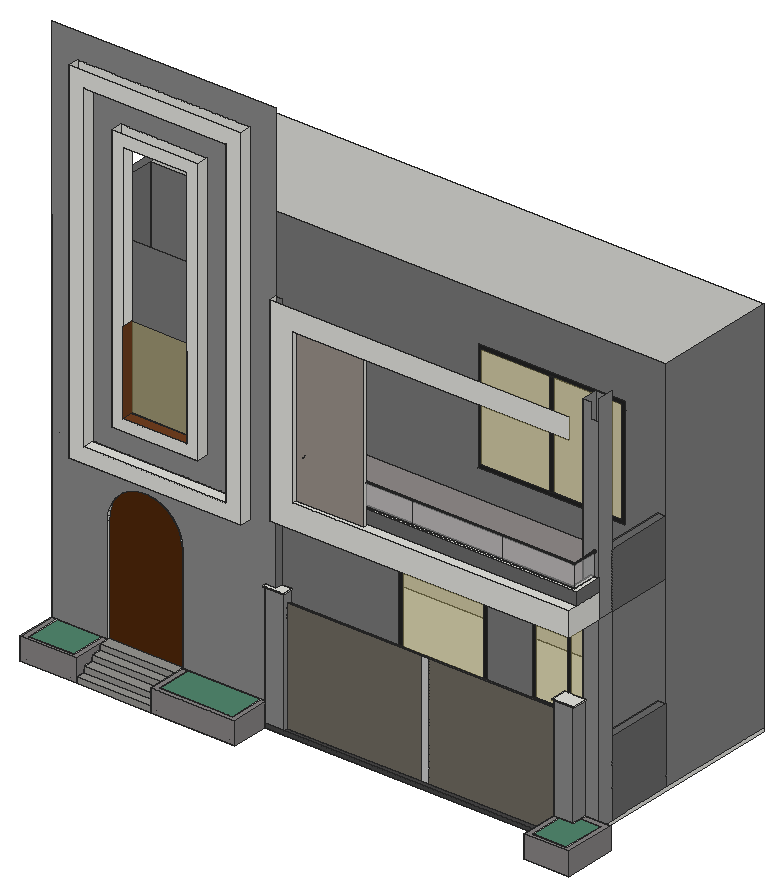
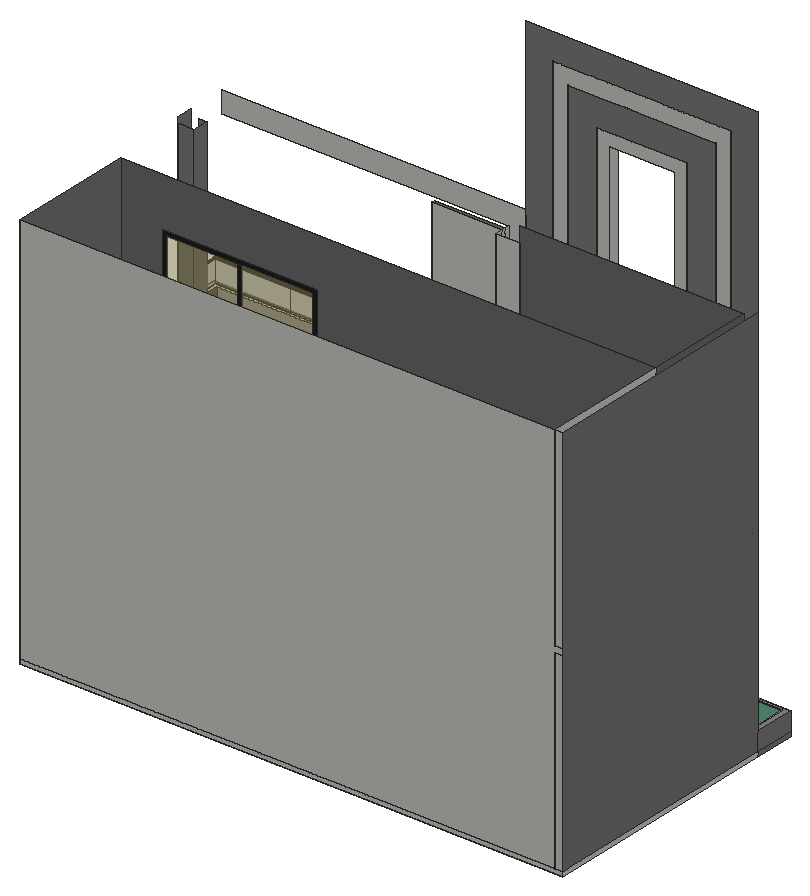
# SketchUp Ruby script. Lengths in inches.
U = 1.inch
M = Sketchup.active_model
def pt(a) = Geom::Point3d.new(a.map { |v| v * U })
def face(e, loops, mat)
  f = e.add_face(loops[0].map { |a| pt(a) })
  loops[1..].each { |l| e.add_face(l.map { |a| pt(a) }).erase! }
  f.material = f.back_material = mat if mat
  f
end
# faces: each face lists its corners as indices into pts; further lists are holes
def faces(e, pts, list, mat = nil) = list.each { |f| face(e, (f[0].is_a?(Array) ? f : [f]).map { |l| l.map { |i| pts[i] } }, mat) }
# xy, xz, yz: faces in a plane at the given z, y or x. An outline is a flat list of corners, or four numbers for a rectangle; further outlines are holes
def ring(l) = l.size == 4 ? [[l[0], l[1]], [l[2], l[1]], [l[2], l[3]], [l[0], l[3]]] : l.each_slice(2).to_a
def flat(e, list, mat, &to3) = list.each { |f| face(e, (f[0].is_a?(Array) ? f : [f]).map { |l| ring(l).map { |u, v| to3.(u, v) } }, mat) }
def xy(e, z, list, mat = nil) = flat(e, list, mat) { |x, y| [x, y, z] }
def xz(e, y, list, mat = nil) = flat(e, list, mat) { |x, z| [x, y, z] }
def yz(e, x, list, mat = nil) = flat(e, list, mat) { |y, z| [x, y, z] }
def lines(e, pts, list) = list.each { |a, b| e.add_line(pt(pts[a]), pt(pts[b])) }
# prism: a flat outline (further loops are holes) pulled along v
def prism(e, loops, v, mat = nil)
  f = face(e, loops, mat); d = Geom::Vector3d.new(v.map { |x| x * U })
  f.pushpull(f.normal.samedirection?(d) ? d.length : -d.length)
end
def box(e, o, s, mat = nil) = prism(e, [[o, [o[0] + s[0], o[1], o[2]], [o[0] + s[0], o[1] + s[1], o[2]], [o[0], o[1] + s[1], o[2]]]], [0, 0, s[2]], mat)
def at(x, y, z, deg = 0) = Geom::Transformation.translation(pt([x, y, z])) * Geom::Transformation.rotation(ORIGIN, Z_AXIS, deg.degrees)
def axes(o, x, y, z) = Geom::Transformation.new([*x, 0, *y, 0, *z, 0, *pt(o).to_a, 1])
def part(name) = M.definitions.add(name)
# library, detail: a bought-in or finely detailed component or shape, given as its bounding box
def library(name, o, s) = part(name).tap { |d| box(d.entities, o, s) }
def detail(e, o, s) = box(e.add_group.entities, o, s)
def put(e, d, t, mat = nil) = e.add_instance(d, t).tap { |i| i.material = mat if mat }
def group(e, t, mat = nil) = e.add_group.tap { |g| g.transformation = t; g.material = mat if mat }.entities
root = M.entities
M.materials.add("[0043_SaddleBrown]").color = [79, 39, 10]
M.materials.add("[0132_LightGray]").color = [137, 137, 137]
M.materials.add("[0133_Gray]").color = [128, 128, 128]
M.materials.add("[0134_DimGray]").color = [105, 105, 105]
M.materials.add("[0136_Charcoal]").color = [35, 35, 35]
M.materials.add("[Brick Tumbled]").color = [135, 132, 132]
M.materials.add("[Carrera Marble]").color = [119, 119, 119]
M.materials.add("[Cladding Stucco White]").color = [200, 200, 200]
M.materials.add("[Cladding Weathered]").color = [111, 105, 96]
M.materials.add("[Diamond Stripes]").color = [153, 144, 137]
M.materials.add("[Granite Dark Gray]").color = [69, 68, 68]
M.materials.add("[Granite Light Gray]").color = [149, 148, 144]
M.materials.add("[Stone Marble]").color = [143, 138, 136]
M.materials.add("[Translucent Glass Gray]").color = [191, 177, 107]
M.materials["[Translucent Glass Gray]"].alpha = 0.5
M.materials.add("[Translucent Glass Gray]1").color = [211, 211, 211]
M.materials["[Translucent Glass Gray]1"].alpha = 0.5
M.materials.add("[Vegetation Ivy Hedera]").color = [81, 134, 109]
M.materials.add("[Wood Cherry Original]").color = [112, 63, 31]
M.materials.add("[Wood Veneer 01]").color = [120, 70, 37]
xy(root,0,[[12,0,192,126],[192,0,432,18],[432,0,702,126],[1629.1875,0,1629.1875,119,1647.1875,119,1647.1875,12,1755.1875,12,1755.1875,149,1692,149,1692,167,1773.1875,167,1773.1875,0],[1647.1875,12,1647.1875,119,1692,119,1692,149,1755.1875,149,1755.1875,12],
  [192,18,432,126],[702,119,702,126,12,126,12,882,1692,882,1692,119]])
xy(root,12,[[30,12,174,126],[450,12,684,126],[1629.1875,119,1692,167],[1666.59,167,1692,222],[1641.1875,222,1692,272.8125],
  [1666.59,272.8125,1692,492],[36,492,1692,882]])
xy(root,12,[[762,119,1629.1875,133.21],[762,133.21,1629.1875,141.23],[762,141.23,1629.1875,141.23,1629.1875,167,1666.59,167,1666.59,222,1641.1875,222,1641.1875,272.8125,1666.59,272.8125,1666.59,492,36,492,36,150,762,150]],"[Granite Dark Gray]")
xy(root,18,[[192,0,432,29.875]],"[Granite Light Gray]")
xy(root,36,[[192,29.875,432,62.5625]],"[Granite Light Gray]")
xy(root,53.25,[[1647.1875,12,1647.1875,119,1692,119,1692,149,1755.1875,149,1755.1875,12]])
xy(root,54,[[192,62.5625,432,94.28]],"[Granite Light Gray]")
xy(root,72,[[12,0,192,0,192,126,174,126,174,12,30,12,30,126,12,126],[432,0,702,0,702,126,684,126,684,12,450,12,450,126,432,126],[1629.1875,0,1773.1875,0,1773.1875,167,1692,167,1692,149,1755.1875,149,1755.1875,12,1647.1875,12,1647.1875,119,1629.1875,119]],"[Brick Tumbled]")
xy(root,72,[[192,94.28,432,132]],"[Granite Light Gray]")
xy(root,72,[[30,12,174,126],[450,12,684,126],[1647.1875,12,1755.1875,12,1755.1875,149,1692,149,1692,119,1647.1875,119]],"[Vegetation Ivy Hedera]")
xy(root,252,[[1666.59,272.8125,1692,492]],"[0134_DimGray]")
xy(root,372,[[762,133.21,1629.1875,141.23]],"[Granite Dark Gray]")
xy(root,405,[[699,116,699,126,702,126,702,119,762,119,762,150,765,150,765,116],[1626.1875,116,1626.1875,167,1629.1875,167,1629.1875,119,1692,119,1692,167,1695,167,1695,116]])
xy(root,408,[[699,116,765,116,765,150,732,150,732,126,699,126],[1626.1875,116,1695,167]])
xy(root,576,[[96,90,648,126]])
xy(root,612,[[824.34,185.95,818.08,186.17,812.09,188,806.77,191.32,802.5,195.9,799.56,201.43,798.15,207.53,798.36,213.8,800.19,219.79,803.51,225.1,808.09,229.375,813.625,232.32,819.73,233.73,825.99,233.51,831.98,231.68,837.3,228.36,841.57,223.78,844.51,218.25,845.92,212.15,845.71,205.88,843.88,199.89,840.56,194.58,835.98,190.3,830.45,187.36],[1112.34,185.95,1106.08,186.17,1100.09,188,1094.77,191.32,1090.5,195.9,1087.56,201.43,1086.15,207.53,1086.36,213.8,1088.19,219.79,1091.51,225.1,1096.09,229.375,1101.625,232.32,1107.73,233.73,1113.99,233.51,1119.98,231.68,1125.3,228.36,1129.57,223.78,1132.51,218.25,1133.92,212.15,1133.71,205.88,1131.88,199.89,1128.56,194.58,1123.98,190.3,1118.45,187.36],[1400.34,185.95,1394.08,186.17,1388.09,188,1382.77,191.32,1378.5,195.9,1375.56,201.43,1374.15,207.53,1374.36,213.8,1376.19,219.79,1379.51,225.1,1384.09,229.375,1389.625,232.32,1395.73,233.73,1401.99,233.51,1407.98,231.68,1413.3,228.36,1417.57,223.78,1420.51,218.25,1421.92,212.15,1421.71,205.88,1419.88,199.89,1416.56,194.58,1411.98,190.3,1406.45,187.36],[824.34,353.95,818.08,354.17,812.09,356,806.77,359.32,802.5,363.9,799.56,369.43,798.15,375.53,798.36,381.8,800.19,387.79,803.51,393.1,808.09,397.375,813.625,400.32,819.73,401.73,825.99,401.51,831.98,399.68,837.3,396.36,841.57,391.78,844.51,386.25,845.92,380.15,845.71,373.88,843.88,367.89,840.56,362.58,835.98,358.3,830.45,355.36],[1112.34,353.95,1106.08,354.17,1100.09,356,1094.77,359.32,1090.5,363.9,1087.56,369.43,1086.15,375.53,1086.36,381.8,1088.19,387.79,1091.51,393.1,1096.09,397.375,1101.625,400.32,1107.73,401.73,1113.99,401.51,1119.98,399.68,1125.3,396.36,1129.57,391.78,1132.51,386.25,1133.92,380.15,1133.71,373.88,1131.88,367.89,1128.56,362.58,1123.98,358.3,1118.45,355.36],
  [1400.34,353.95,1394.08,354.17,1388.09,356,1382.77,359.32,1378.5,363.9,1375.56,369.43,1374.15,375.53,1374.36,381.8,1376.19,387.79,1379.51,393.1,1384.09,397.375,1389.625,400.32,1395.73,401.73,1401.99,401.51,1407.98,399.68,1413.3,396.36,1417.57,391.78,1420.51,386.25,1421.92,380.15,1421.71,373.88,1419.88,367.89,1416.56,362.58,1411.98,358.3,1406.45,355.36]])
xy(root,612,[[[732,102,732,150,36,150,36,492,1692,492,1692,272.8125,1641.1875,272.8125,1641.1875,222,1692,222,1692,102],[1112.34,353.95,1118.45,355.36,1123.98,358.3,1128.56,362.58,1131.88,367.89,1133.71,373.88,1133.92,380.15,1132.51,386.25,1129.57,391.78,1125.3,396.36,1119.98,399.68,1113.99,401.51,1107.73,401.73,1101.625,400.32,1096.09,397.375,1091.51,393.1,1088.19,387.79,1086.36,381.8,1086.15,375.53,1087.56,369.43,1090.5,363.9,1094.77,359.32,1100.09,356,1106.08,354.17],[1400.34,353.95,1406.45,355.36,1411.98,358.3,1416.56,362.58,1419.88,367.89,1421.71,373.88,1421.92,380.15,1420.51,386.25,1417.57,391.78,1413.3,396.36,1407.98,399.68,1401.99,401.51,1395.73,401.73,1389.625,400.32,1384.09,397.375,1379.51,393.1,1376.19,387.79,1374.36,381.8,1374.15,375.53,1375.56,369.43,1378.5,363.9,1382.77,359.32,1388.09,356,1394.08,354.17],[824.34,185.95,830.45,187.36,835.98,190.3,840.56,194.58,843.88,199.89,845.71,205.88,845.92,212.15,844.51,218.25,841.57,223.78,837.3,228.36,831.98,231.68,825.99,233.51,819.73,233.73,813.625,232.32,808.09,229.375,803.51,225.1,800.19,219.79,798.36,213.8,798.15,207.53,799.56,201.43,802.5,195.9,806.77,191.32,812.09,188,818.08,186.17],[824.34,353.95,830.45,355.36,835.98,358.3,840.56,362.58,843.88,367.89,845.71,373.88,845.92,380.15,844.51,386.25,841.57,391.78,837.3,396.36,831.98,399.68,825.99,401.51,819.73,401.73,813.625,400.32,808.09,397.375,803.51,393.1,800.19,387.79,798.36,381.8,798.15,375.53,799.56,369.43,802.5,363.9,806.77,359.32,812.09,356,818.08,354.17],[1112.34,185.95,1118.45,187.36,1123.98,190.3,1128.56,194.58,1131.88,199.89,1133.71,205.88,1133.92,212.15,1132.51,218.25,1129.57,223.78,1125.3,228.36,1119.98,231.68,1113.99,233.51,1107.73,233.73,1101.625,232.32,1096.09,229.375,1091.51,225.1,1088.19,219.79,1086.36,213.8,1086.15,207.53,1087.56,201.43,1090.5,195.9,1094.77,191.32,1100.09,188,1106.08,186.17],[1400.34,185.95,1406.45,187.36,1411.98,190.3,1416.56,194.58,1419.88,199.89,1421.71,205.88,1421.92,212.15,1420.51,218.25,1417.57,223.78,1413.3,228.36,1407.98,231.68,1401.99,233.51,1395.73,233.73,1389.625,232.32,1384.09,229.375,1379.51,225.1,1376.19,219.79,1374.36,213.8,1374.15,207.53,1375.56,201.43,1378.5,195.9,1382.77,191.32,1388.09,188,1394.08,186.17]]],"[Wood Veneer 01]")
xy(root,624,[[144,90,600,126]])
xy(root,630,[[36,150,1666.59,150,1666.59,222,1641.1875,222,1641.1875,272.8125,1666.59,272.8125,1666.59,492,36,492]],"[Stone Marble]")
xy(root,690,[[804,102,1692,102,1692,133,804,133,804,126,1021.625,126,1021.625,115.125,804,115.125],[804,115.125,1021.625,126],[732,126,804,150]])
xy(root,712.57,[[232.57,90,511.43,126]])
xy(root,732,[[804,133,1692,133,1692,222,1679.3,222,1679.3,141.5,804,141.5],[804,141.5,1679.3,141.5,1679.3,222,1666.59,222,1666.59,150,804,150]])
xy(root,748.57,[[268.57,90,475.43,126]],"[Wood Cherry Original]")
xy(root,792,[[1666.59,272.8125,1692,492]],"[0134_DimGray]")
xz(root,0,[[12,0,192,72],[432,0,702,72],[1629.1875,0,1773.1875,72]],"[Brick Tumbled]")
xz(root,0,[[192,0,432,18]],"[Granite Light Gray]")
xz(root,12,[[1647.1875,0,1755.1875,53.25],[30,12,174,72],[450,12,684,72],[1647.1875,53.25,1755.1875,72]])
xz(root,29.875,[[192,18,432,36]],"[Granite Light Gray]")
xz(root,62.5625,[[192,36,432,54]],"[Granite Light Gray]")
xz(root,90,[[[96,576,648,1704],[144,624,600,1656]],[[232.57,712.57,511.43,1567.43],[268.57,748.57,475.43,1531.43]]])
xz(root,94.28,[[192,54,432,72]],"[Granite Light Gray]")
xz(root,102,[[732,612,1692,612,1692,690,804,690,804,1182,1692,1182,1692,1248,732,1248]])
xz(root,115.125,[[804,690,1021.625,1182]],"[Diamond Stripes]")
xz(root,116,[[699,405,765,408],[1626.1875,405,1695,408]])
xz(root,119,[[1629.1875,0,1647.1875,12],[1647.1875,0,1692,12],[1629.1875,12,1647.1875,72],[1647.1875,12,1692,53.25],[1647.1875,53.25,1692,72]])
xz(root,119,[[702,12,762,405],[1629.1875,72,1692,405]],"[0132_LightGray]")
xz(root,119,[[702,0,1629.1875,12]],"[Granite Dark Gray]")
xz(root,126,[[12,0,12,72,30,72,30,12,174,12,174,72,192,72,192,0],[192,0,432,18],[432,0,432,72,450,72,450,12,684,12,684,72,702,72,702,0],[30,12,36,72],[36,12,174,72],
  [450,12,684,72],[192,18,432,36],[192,36,432,54],[699,405,702,408],[[96,576,648,1704],[144,624,600,1656]],
  [804,690,1021.625,1182],[[232.57,712.57,511.43,1567.43],[268.57,748.57,475.43,1531.43]]])
xz(root,126,[[[12,72,192,72,192,412.67,193.01,428.18,196.01,443.44,200.96,458.17,207.78,472.15,216.34,485.12,226.51,496.88,238.12,507.23,250.97,515.98,264.84,523.01,279.55,528,285.88,529.79,292.34,531.04,298.86,531.94,305.42,532.49,312,532.67,318.58,532.49,325.14,531.94,331.66,531.04,338.12,529.79,344.45,528,359.16,523.01,373.03,515.98,385.88,507.23,397.49,496.88,407.66,485.12,416.22,472.15,423.04,458.17,427.99,443.44,430.99,428.18,432,412.67,432,72,702,72,702,405,699,405,699,408,732,408,732,1788,12,1788],[96,576,648,1704]],[[144,624,600,1656],[232.57,712.57,511.43,1567.43]]],"[0132_LightGray]")
xz(root,126,[[268.57,748.57,475.43,1012.57]],"[Translucent Glass Gray]")
xz(root,132,[[192,72,432,72,432,412.67,430.99,428.18,427.99,443.44,423.04,458.17,416.22,472.15,407.66,485.12,397.49,496.88,385.88,507.23,373.03,515.98,359.16,523.01,344.45,528,338.12,529.79,331.66,531.04,325.14,531.94,318.58,532.49,312,532.67,305.42,532.49,298.86,531.94,292.34,531.04,285.88,529.79,279.55,528,264.84,523.01,250.97,515.98,238.12,507.23,226.51,496.88,216.34,485.12,207.78,472.15,200.96,458.17,196.01,443.44,193.01,428.18,192,412.67]],"[0043_SaddleBrown]")
xz(root,133,[[804,690,1692,732]],"[0134_DimGray]")
xz(root,133.21,[[1195.59,12,1216.73,372]],"[Cladding Stucco White]")
xz(root,133.21,[[762,12,1195.59,372],[1216.73,12,1629.1875,372]],"[Cladding Weathered]")
xz(root,141.23,[[762,12,1629.1875,372]],"[Cladding Weathered]")
xz(root,141.5,[[804,801,1679.3,804]])
xz(root,141.5,[[804,732,1158.38,801],[1158.38,732,1446.38,801],[1446.38,732,1679.3,801]],"[Translucent Glass Gray]1")
xz(root,149,[[1692,0,1755.1875,53.25],[1692,53.25,1755.1875,72]])
xz(root,150,[[762,405,765,408],[732,630,732,690,804,690,804,732,1666.59,732,1666.59,630],[732,690,804,1182]])
xz(root,150,[[732,12,762,408]],"[0132_LightGray]")
xz(root,150,[[36,12,732,612],[36,630,732,1230]],"[Carrera Marble]")
xz(root,167,[[1692,0,1773.1875,72],[1626.1875,405,1629.1875,408],[1692,405,1695,408]])
xz(root,167,[[1629.1875,12,1692,408]],"[0132_LightGray]")
xz(root,222,[[1666.59,630,1692,690],[1666.59,690,1692,732],[1679.3,801,1678.98,801.02,1678.67,801.07,1678.37,801.15,1678.08,801.26,1677.8,801.4,1677.53,801.57,1677.29,801.77,1677.07,801.99,1676.87,802.24,1676.7,802.5,1676.56,802.78,1676.44,803.07,1676.36,803.375,1676.3125,803.6875,1676.3,804,1676.3125,804.3125,1676.36,804.625,1676.44,804.93,1676.56,805.22,1676.7,805.5,1676.87,805.76,1677.07,806.01,1677.29,806.23,1677.53,806.43,1677.8,806.6,1678.08,806.74,1678.37,806.85,1678.67,806.93,1678.98,806.98,1679.3,807,1679.61,806.98,1679.92,806.93,1680.22,806.85,1680.52,806.74,1680.8,806.6,1681.06,806.43,1681.3,806.23,1681.53,806.01,1681.72,805.76,1681.89,805.5,1682.04,805.22,1682.15,804.93,1682.23,804.625,1682.28,804.3125,1682.3,804,1682.28,803.6875,1682.23,803.375,1682.15,803.07,1682.04,802.78,1681.89,802.5,1681.72,802.24,1681.53,801.99,1681.3,801.77,1681.06,801.57,1680.8,801.4,1680.52,801.26,1680.22,801.15,1679.92,801.07,1679.61,801.02]])
xz(root,222,[[1641.1875,12,1692,612],[[1641.1875,630,1666.59,630,1666.59,732,1692,732,1692,1182,1666.59,1182,1666.59,1230,1641.1875,1230],[1679.3,801,1678.98,801.02,1678.67,801.07,1678.37,801.15,1678.08,801.26,1677.8,801.4,1677.53,801.57,1677.29,801.77,1677.07,801.99,1676.87,802.24,1676.7,802.5,1676.56,802.78,1676.44,803.07,1676.36,803.375,1676.3125,803.6875,1676.3,804,1676.3125,804.3125,1676.36,804.625,1676.44,804.93,1676.56,805.22,1676.7,805.5,1676.87,805.76,1677.07,806.01,1677.29,806.23,1677.53,806.43,1677.8,806.6,1678.08,806.74,1678.37,806.85,1678.67,806.93,1678.98,806.98,1679.3,807,1679.61,806.98,1679.92,806.93,1680.22,806.85,1680.52,806.74,1680.8,806.6,1681.06,806.43,1681.3,806.23,1681.53,806.01,1681.72,805.76,1681.89,805.5,1682.04,805.22,1682.15,804.93,1682.23,804.625,1682.28,804.3125,1682.3,804,1682.28,803.6875,1682.23,803.375,1682.15,803.07,1682.04,802.78,1681.89,802.5,1681.72,802.24,1681.53,801.99,1681.3,801.77,1681.06,801.57,1680.8,801.4,1680.52,801.26,1680.22,801.15,1679.92,801.07,1679.61,801.02]]],"[0132_LightGray]")
xz(root,272.8125,[[1666.59,12,1692,252],[1666.59,630,1692,732],[1666.59,732,1692,792]])
xz(root,272.8125,[[1641.1875,12,1641.1875,612,1692,612,1692,252,1666.59,252,1666.59,12],[1641.1875,630,1641.1875,1230,1692,1230,1692,792,1666.59,792,1666.59,630]],"[0132_LightGray]")
xz(root,492,[[1666.59,12,1692,252],[1666.59,630,1692,732],[1666.59,732,1692,792]])
xz(root,492,[[[831.57,12,1120.32,419.6875],[846.31,26.74,1105.58,404.95]],[[1261.8,110.58,1499.8,416.95],[1273.8,122.58,1374.8,404.95],[1386.8,122.58,1487.8,404.95]],[[1086.33,718.2,1561.39,1076.45],[1098.33,730.2,1549.39,1064.45]],[1317.86,730.2,1329.86,1064.45]],"[0136_Charcoal]")
xz(root,492,[[[36,12,831.57,12,831.57,419.6875,1120.32,419.6875,1120.32,12,1666.59,12,1666.59,252,1692,252,1692,612,36,612],[1261.8,110.58,1499.8,416.95]],[[36,630,1666.59,630,1666.59,792,1692,792,1692,1230,36,1230],[1086.33,718.2,1561.39,1076.45]]],"[Carrera Marble]")
xz(root,492,[[846.31,26.74,1105.58,404.95],[1273.8,122.58,1374.8,404.95],[1386.8,122.58,1487.8,404.95],[1098.33,730.2,1317.86,1064.45],[1329.86,730.2,1549.39,1064.45]],"[Translucent Glass Gray]")
xz(root,882,[[12,0,1692,12],[12,12,36,612],[36,12,36,612,12,612,12,630,36,630,36,1230,1692,1230,1692,12],[12,630,36,1230]])
yz(root,12,[[126,0,882,12]])
yz(root,12,[[126,12,882,1230]],"[0133_Gray]")
yz(root,12,[[0,0,126,12],[0,12,126,72]],"[Brick Tumbled]")
yz(root,30,[[12,12,126,72]])
yz(root,36,[[492,12,882,612],[492,630,882,1230]])
yz(root,36,[[150,12,492,612],[150,630,492,1230]],"[Carrera Marble]")
yz(root,96,[[90,576,126,1704]])
yz(root,144,[[90,624,126,1656]])
yz(root,174,[[12,12,126,72]])
yz(root,192,[[0,0,126,18],[29.875,18,126,36],[62.5625,36,126,54],[94.28,54,126,72],[126,72,132,412.67]])
yz(root,192,[[0,18,29.875,18,29.875,36,62.5625,36,62.5625,54,94.28,54,94.28,72,0,72]],"[Brick Tumbled]")
yz(root,232.57,[[90,712.57,126,1567.43]])
yz(root,268.57,[[90,748.57,126,1012.57]],"[Wood Cherry Original]")
yz(root,432,[[0,0,126,18],[29.875,18,126,36],[62.5625,36,126,54],[94.28,54,126,72],[126,72,132,412.67]])
yz(root,432,[[0,18,0,72,94.28,72,94.28,54,62.5625,54,62.5625,36,29.875,36,29.875,18]],"[Brick Tumbled]")
yz(root,450,[[12,12,126,72]])
yz(root,475.43,[[90,748.57,126,1012.57]],"[Wood Cherry Original]")
yz(root,511.43,[[90,712.57,126,1567.43]])
yz(root,600,[[90,624,126,1656]])
yz(root,648,[[90,576,126,1704]])
yz(root,684,[[12,12,126,72]])
yz(root,699,[[116,405,119,408],[119,405,126,408]])
yz(root,702,[[119,0,126,72],[119,72,126,405]])
yz(root,702,[[0,0,119,72]],"[Brick Tumbled]")
yz(root,732,[[102,612,126,1248],[126,630,150,690],[126,690,150,1182]])
yz(root,732,[[126,408,150,612]],"[Carrera Marble]")
yz(root,762,[[119,12,133.21,12,133.21,372,141.23,372,141.23,12,150,12,150,405,119,405]],"[0132_LightGray]")
yz(root,762,[[133.21,12,141.23,372]],"[Granite Dark Gray]")
yz(root,765,[[116,405,150,408]])
yz(root,804,[[102,690,115.125,1182],[115.125,690,126,1182],[[126,690,133,690,133,732,150,732,150,1182,126,1182],[141.5,801,141.1875,801.02,140.875,801.07,140.57,801.15,140.28,801.26,140,801.4,139.74,801.57,139.49,801.77,139.27,801.99,139.07,802.24,138.9,802.5,138.76,802.78,138.65,803.07,138.57,803.375,138.52,803.6875,138.5,804,138.52,804.3125,138.57,804.625,138.65,804.93,138.76,805.22,138.9,805.5,139.07,805.76,139.27,806.01,139.49,806.23,139.74,806.43,140,806.6,140.28,806.74,140.57,806.85,140.875,806.93,141.1875,806.98,141.5,807,141.8125,806.98,142.125,806.93,142.43,806.85,142.72,806.74,143,806.6,143.26,806.43,143.51,806.23,143.73,806.01,143.93,805.76,144.1,805.5,144.24,805.22,144.35,804.93,144.43,804.625,144.48,804.3125,144.5,804,144.48,803.6875,144.43,803.375,144.35,803.07,144.24,802.78,144.1,802.5,143.93,802.24,143.73,801.99,143.51,801.77,143.26,801.57,143,801.4,142.72,801.26,142.43,801.15,142.125,801.07,141.8125,801.02]],[133,690,150,732]])
yz(root,1021.625,[[115.125,690,126,1182]])
yz(root,1626.1875,[[116,405,167,408]])
yz(root,1629.1875,[[119,12,119,405,167,405,167,12,141.23,12,141.23,372,133.21,372,133.21,12]],"[0132_LightGray]")
yz(root,1629.1875,[[0,0,119,72]],"[Brick Tumbled]")
yz(root,1629.1875,[[133.21,12,141.23,372]],"[Granite Dark Gray]")
yz(root,1641.1875,[[222,12,272.8125,612],[222,630,272.8125,1230]],"[0132_LightGray]")
yz(root,1647.1875,[[12,0,119,53.25],[12,53.25,119,72]])
yz(root,1666.59,[[272.8125,12,492,252],[150,630,222,732],[272.8125,630,492,792]],"[0134_DimGray]")
yz(root,1679.3,[[141.5,801,222,804]])
yz(root,1679.3,[[141.5,732,222,801]],"[Translucent Glass Gray]1")
yz(root,1692,[[119,0,149,12],[149,0,167,12],[167,0,882,12],[119,12,149,53.25],[149,12,167,72],
  [119,53.25,149,72],[102,612,222,690]])
yz(root,1692,[[222,12,272.8125,612],[119,72,167,405],[222,612,272.8125,1248]],"[0132_LightGray]")
yz(root,1692,[[492,12,882,1230]],"[0133_Gray]")
yz(root,1692,[[272.8125,12,492,252],[272.8125,612,492,792],[133,690,222,732]],"[0134_DimGray]")
yz(root,1695,[[116,405,167,408]])
yz(root,1755.1875,[[12,0,149,53.25],[12,53.25,149,72]])
yz(root,1773.1875,[[0,0,167,72]],"[Brick Tumbled]")
p = [[193.01,126,428.18],[192,126,412.67],[192,132,412.67],[193.01,132,428.18],[432,126,412.67],[430.99,126,428.18],
  [430.99,132,428.18],[432,132,412.67],[196.01,126,443.44],[196.01,132,443.44],[427.99,126,443.44],[427.99,132,443.44],
  [200.96,126,458.17],[200.96,132,458.17],[423.04,126,458.17],[423.04,132,458.17],[207.78,126,472.15],[207.78,132,472.15],
  [416.22,126,472.15],[416.22,132,472.15],[216.34,126,485.12],[216.34,132,485.12],[407.66,126,485.12],[407.66,132,485.12],
  [226.51,126,496.88],[226.51,132,496.88],[397.49,126,496.88],[397.49,132,496.88],[238.12,126,507.23],[238.12,132,507.23],
  [385.88,126,507.23],[385.88,132,507.23],[250.97,126,515.98],[250.97,132,515.98],[373.03,126,515.98],[373.03,132,515.98],
  [264.84,126,523.01],[264.84,132,523.01],[359.16,126,523.01],[359.16,132,523.01],[279.55,126,528],[279.55,132,528],
  [344.45,126,528],[344.45,132,528],[285.88,126,529.79],[285.88,132,529.79],[338.12,126,529.79],[338.12,132,529.79],
  [292.34,126,531.04],[292.34,132,531.04],[331.66,126,531.04],[331.66,132,531.04],[298.86,126,531.94],[298.86,132,531.94],
  [325.14,126,531.94],[325.14,132,531.94],[305.42,126,532.49],[305.42,132,532.49],[318.58,126,532.49],[318.58,132,532.49],
  [312,126,532.67],[312,132,532.67],[1679.61,141.1875,801.02],[1679.92,140.875,801.07],[804,140.875,801.07],[804,141.1875,801.02],
  [1679.61,222,801.02],[1679.92,222,801.07],[1679.3,141.5,801],[804,141.5,801],[1158.38,141.5,801],[1446.38,141.5,801],
  [1679.3,222,801],[1678.98,141.8125,801.02],[804,141.8125,801.02],[1678.98,222,801.02],[1678.67,142.125,801.07],[804,142.125,801.07],
  [1678.67,222,801.07],[1680.22,140.57,801.15],[1680.52,140.28,801.26],[804,140.28,801.26],[804,140.57,801.15],[1680.22,222,801.15],
  [1680.52,222,801.26],[1678.37,142.43,801.15],[804,142.43,801.15],[1678.37,222,801.15],[1678.08,142.72,801.26],[804,142.72,801.26],
  [1678.08,222,801.26],[1680.8,140,801.4],[804,140,801.4],[1680.8,222,801.4],[1677.8,143,801.4],[804,143,801.4],
  [1677.8,222,801.4],[1681.06,139.74,801.57],[804,139.74,801.57],[1681.06,222,801.57],[1677.53,143.26,801.57],[804,143.26,801.57],
  [1677.53,222,801.57],[1681.3,139.49,801.77],[804,139.49,801.77],[1681.3,222,801.77],[1677.29,143.51,801.77],[804,143.51,801.77],
  [1677.29,222,801.77],[1681.53,139.27,801.99],[804,139.27,801.99],[1681.53,222,801.99],[1677.07,143.73,801.99],[804,143.73,801.99],
  [1677.07,222,801.99],[1681.72,139.07,802.24],[804,139.07,802.24],[1681.72,222,802.24],[1676.87,143.93,802.24],[804,143.93,802.24],
  [1676.87,222,802.24],[1681.89,138.9,802.5],[804,138.9,802.5],[1681.89,222,802.5],[1676.7,144.1,802.5],[804,144.1,802.5],
  [1676.7,222,802.5],[1682.04,138.76,802.78],[804,138.76,802.78],[1682.04,222,802.78],[1676.56,144.24,802.78],[804,144.24,802.78],
  [1676.56,222,802.78],[1682.15,138.65,803.07],[804,138.65,803.07],[1682.15,222,803.07],[1676.44,144.35,803.07],[804,144.35,803.07],
  [1676.44,222,803.07],[1682.23,138.57,803.375],[804,138.57,803.375],[1682.23,222,803.375],[1676.36,144.43,803.375],[804,144.43,803.375],
  [1676.36,222,803.375],[1682.28,138.52,803.6875],[804,138.52,803.6875],[1682.28,222,803.6875],[1676.3125,144.48,803.6875],[804,144.48,803.6875],
  [1676.3125,222,803.6875],[1682.3,138.5,804],[804,138.5,804],[1682.3,222,804],[1676.3,144.5,804],[804,144.5,804],
  [1676.3,222,804],[1682.28,138.52,804.3125],[804,138.52,804.3125],[1682.28,222,804.3125],[1676.3125,144.48,804.3125],[804,144.48,804.3125],
  [1676.3125,222,804.3125],[1682.23,138.57,804.625],[804,138.57,804.625],[1682.23,222,804.625],[1676.36,144.43,804.625],[804,144.43,804.625],
  [1676.36,222,804.625],[1682.15,138.65,804.93],[804,138.65,804.93],[1682.15,222,804.93],[1676.44,144.35,804.93],[804,144.35,804.93],
  [1676.44,222,804.93],[1682.04,138.76,805.22],[804,138.76,805.22],[1682.04,222,805.22],[1676.56,144.24,805.22],[804,144.24,805.22],
  [1676.56,222,805.22],[1681.89,138.9,805.5],[804,138.9,805.5],[1681.89,222,805.5],[1676.7,144.1,805.5],[804,144.1,805.5],
  [1676.7,222,805.5],[1681.72,139.07,805.76],[804,139.07,805.76],[1681.72,222,805.76],[1676.87,143.93,805.76],[804,143.93,805.76],
  [1676.87,222,805.76],[1681.53,139.27,806.01],[804,139.27,806.01],[1681.53,222,806.01],[1677.07,143.73,806.01],[804,143.73,806.01],
  [1677.07,222,806.01],[1681.3,139.49,806.23],[804,139.49,806.23],[1681.3,222,806.23],[1677.29,143.51,806.23],[804,143.51,806.23],
  [1677.29,222,806.23],[1681.06,139.74,806.43],[804,139.74,806.43],[1681.06,222,806.43],[1677.53,143.26,806.43],[804,143.26,806.43],
  [1677.53,222,806.43],[1680.8,140,806.6],[804,140,806.6],[1680.8,222,806.6],[1677.8,143,806.6],[804,143,806.6],
  [1677.8,222,806.6],[1680.52,140.28,806.74],[804,140.28,806.74],[1680.52,222,806.74],[1678.08,142.72,806.74],[804,142.72,806.74],
  [1678.08,222,806.74],[1680.22,140.57,806.85],[804,140.57,806.85],[1680.22,222,806.85],[1678.37,142.43,806.85],[804,142.43,806.85],
  [1678.37,222,806.85],[1679.92,140.875,806.93],[804,140.875,806.93],[1679.92,222,806.93],[1679.61,141.1875,806.98],[804,141.1875,806.98],
  [1679.61,222,806.98],[1678.98,141.8125,806.98],[1678.67,142.125,806.93],[804,142.125,806.93],[804,141.8125,806.98],[1678.98,222,806.98],
  [1678.67,222,806.93],[1679.3,141.5,807],[804,141.5,807],[1679.3,222,807],[36,126,12],[36,150,12],
  [36,126,612],[36,150,612],[36,150,630],[12,150,630],[804,133,688.5625],[804,126,688.5625],
  [1692,133,688.5625],[804,133,690],[732,126,12],[732,150,12],[450,12,12],[450,0,12],
  [684,12,12],[684,0,12],[174,12,12],[174,0,12],[30,12,12],[30,0,12]]
faces(root,p,[[0,1,2,3],[4,5,6,7],[8,0,3,9],[5,10,11,6],[12,8,9,13],[10,14,15,11],[16,12,13,17],[14,18,19,15],
  [20,16,17,21],[18,22,23,19],[24,20,21,25],[22,26,27,23],[28,24,25,29],[26,30,31,27],[32,28,29,33],[30,34,35,31],
  [36,32,33,37],[34,38,39,35],[40,36,37,41],[38,42,43,39],[44,40,41,45],[42,46,47,43],[48,44,45,49],[46,50,51,47],
  [52,48,49,53],[50,54,55,51],[56,52,53,57],[54,58,59,55],[60,56,57,61],[58,60,61,59],[62,63,64,65],[66,67,63,62],
  [68,62,65,69,70,71],[72,66,62,68],[73,68,71,70,69,74],[75,72,68,73],[76,73,74,77],[78,75,73,76],[79,80,81,82],[83,84,80,79],
  [63,79,82,64],[67,83,79,63],[85,76,77,86],[87,78,76,85],[88,85,86,89],[90,87,85,88],[80,91,92,81],[84,93,91,80],
  [94,88,89,95],[96,90,88,94],[91,97,98,92],[93,99,97,91],[100,94,95,101],[102,96,94,100],[97,103,104,98],[99,105,103,97],
  [106,100,101,107],[108,102,100,106],[103,109,110,104],[105,111,109,103],[112,106,107,113],[114,108,106,112],[109,115,116,110],[111,117,115,109],
  [118,112,113,119],[120,114,112,118],[115,121,122,116],[117,123,121,115],[124,118,119,125],[126,120,118,124],[121,127,128,122],[123,129,127,121],
  [130,124,125,131],[132,126,124,130],[127,133,134,128],[129,135,133,127],[136,130,131,137],[138,132,130,136],[133,139,140,134],[135,141,139,133],
  [142,136,137,143],[144,138,136,142],[139,145,146,140],[141,147,145,139],[148,142,143,149],[150,144,142,148],[145,151,152,146],[147,153,151,145],
  [154,148,149,155],[156,150,148,154],[151,157,158,152],[153,159,157,151],[160,154,155,161],[162,156,154,160],[157,163,164,158],[159,165,163,157],
  [166,160,161,167],[168,162,160,166],[163,169,170,164],[165,171,169,163],[172,166,167,173],[174,168,166,172],[169,175,176,170],[171,177,175,169],
  [178,172,173,179],[180,174,172,178],[175,181,182,176],[177,183,181,175],[184,178,179,185],[186,180,178,184],[181,187,188,182],[183,189,187,181],
  [190,184,185,191],[192,186,184,190],[187,193,194,188],[189,195,193,187],[196,190,191,197],[198,192,190,196],[193,199,200,194],[195,201,199,193],
  [202,196,197,203],[204,198,196,202],[199,205,206,200],[201,207,205,199],[208,202,203,209],[210,204,202,208],[205,211,212,206],[207,213,211,205],
  [214,208,209,215],[216,210,208,214],[211,217,218,212],[213,219,217,211],[220,214,215,221],[222,216,214,220],[217,223,224,218],[219,225,223,217],
  [226,220,221,227],[228,222,220,226],[223,229,230,224],[225,231,229,223],[229,232,233,230],[231,234,232,229],[235,236,237,238],[239,240,236,235],
  [236,226,227,237],[240,228,226,236],[232,241,242,233],[234,243,241,232],[241,235,238,242],[243,239,235,241]])
lines(root,p,[[244,245],[246,247],[248,249],[250,251],[250,252],[253,250],[254,255],[256,257],[258,259],[260,261],[262,263]])
